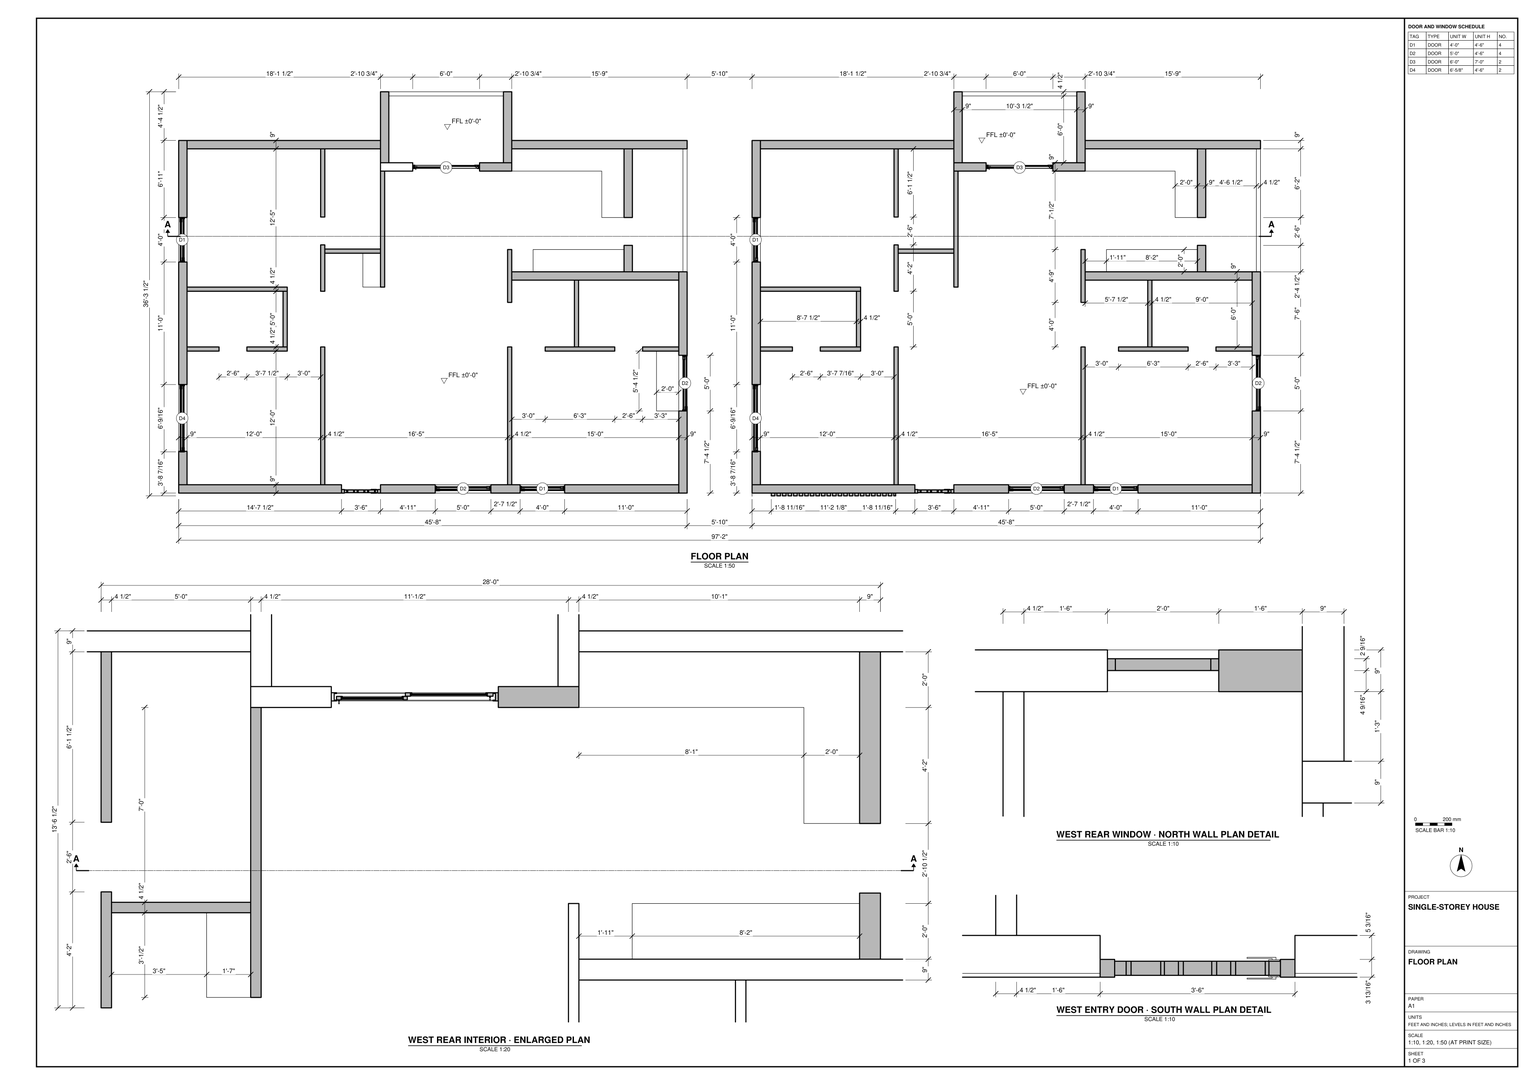
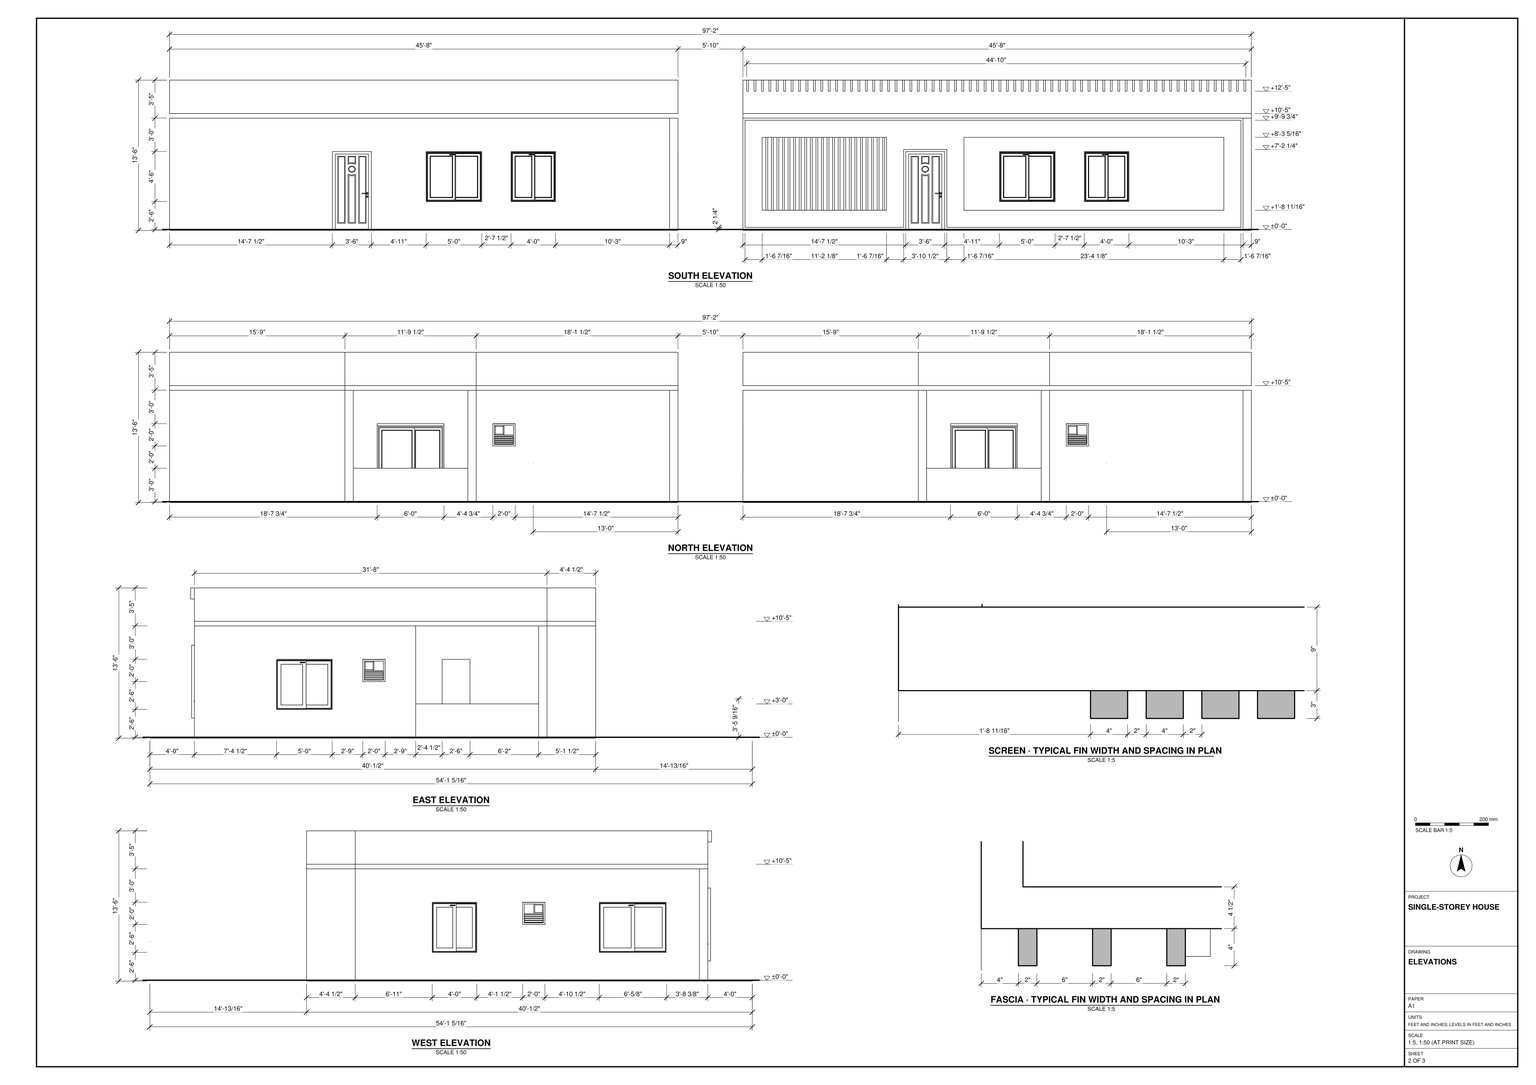
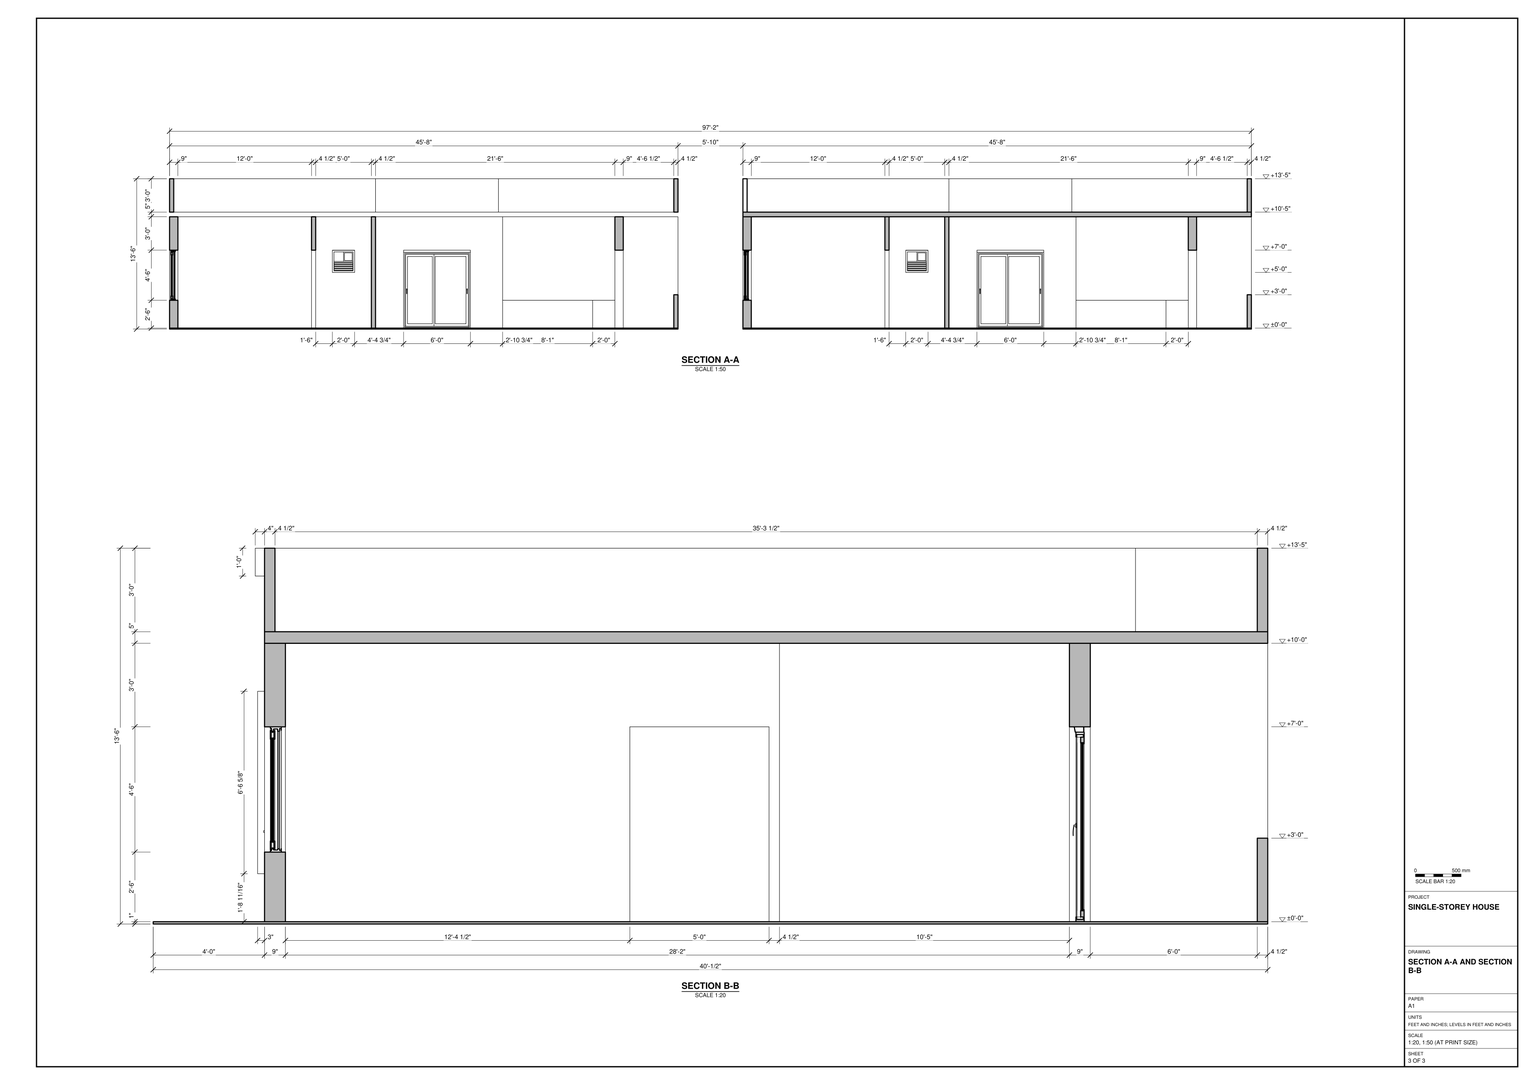
Build a SketchUp model from task_files/diagram_01.pdf. Work in feet and inches. Set the finished floor of both blocks at ±0'-0". The overall model extents are 97'-2" east to west, 54'-1 5/16" north to south and 13'-6" vertically.

Lay out the blocks side by side with their entrances facing south. Each block is 45'-8" wide, with a 5'-10" clear gap between them. Follow the floor plan for the exterior walls, thinner interior partitions, passages and projecting rear bays. Use the enlarged rear plan to place the built-in work surfaces and their returns. Model the floor slabs, flat roof and parapets as shown in section.

Fit the entry doors, framed windows, rear sliding doors and small ventilators at the positions and heights shown. Keep the western block's south elevation plain. On the eastern block, model the screen to the left of the entrance, the surround at the pair of windows and the fins along the fascia. Use the separate plan details for the screen and fascia rather than giving both the same spacing.

Keep shell elements such as walls, slabs and roof, and each furniture or joinery piece, in separate groups or components. Use components for repeated parts. Decor and loose items may be any suitable library components. Save one SketchUp model as output_files/two_single_storey_house_blocks_with_distinct_facades.skp.

# SketchUp Ruby script. Lengths in inches.
U = 1.inch
M = Sketchup.active_model
def pt(a) = Geom::Point3d.new(a.map { |v| v * U })
def face(e, loops, mat)
  f = e.add_face(loops[0].map { |a| pt(a) })
  loops[1..].each { |l| e.add_face(l.map { |a| pt(a) }).erase! }
  f.material = f.back_material = mat if mat
  f
end
# faces: each face lists its corners as indices into pts; further lists are holes
def faces(e, pts, list, mat = nil) = list.each { |f| face(e, (f[0].is_a?(Array) ? f : [f]).map { |l| l.map { |i| pts[i] } }, mat) }
# xy, xz, yz: faces in a plane at the given z, y or x. An outline is a flat list of corners, or four numbers for a rectangle; further outlines are holes
def ring(l) = l.size == 4 ? [[l[0], l[1]], [l[2], l[1]], [l[2], l[3]], [l[0], l[3]]] : l.each_slice(2).to_a
def flat(e, list, mat, &to3) = list.each { |f| face(e, (f[0].is_a?(Array) ? f : [f]).map { |l| ring(l).map { |u, v| to3.(u, v) } }, mat) }
def xy(e, z, list, mat = nil) = flat(e, list, mat) { |x, y| [x, y, z] }
def xz(e, y, list, mat = nil) = flat(e, list, mat) { |x, z| [x, y, z] }
def yz(e, x, list, mat = nil) = flat(e, list, mat) { |y, z| [x, y, z] }
def lines(e, pts, list) = list.each { |a, b| e.add_line(pt(pts[a]), pt(pts[b])) }
# prism: a flat outline (further loops are holes) pulled along v
def prism(e, loops, v, mat = nil)
  f = face(e, loops, mat); d = Geom::Vector3d.new(v.map { |x| x * U })
  f.pushpull(f.normal.samedirection?(d) ? d.length : -d.length)
end
def box(e, o, s, mat = nil) = prism(e, [[o, [o[0] + s[0], o[1], o[2]], [o[0] + s[0], o[1] + s[1], o[2]], [o[0], o[1] + s[1], o[2]]]], [0, 0, s[2]], mat)
def at(x, y, z, deg = 0) = Geom::Transformation.translation(pt([x, y, z])) * Geom::Transformation.rotation(ORIGIN, Z_AXIS, deg.degrees)
def axes(o, x, y, z) = Geom::Transformation.new([*x, 0, *y, 0, *z, 0, *pt(o).to_a, 1])
def part(name) = M.definitions.add(name)
# library, detail: a bought-in or finely detailed component or shape, given as its bounding box
def library(name, o, s) = part(name).tap { |d| box(d.entities, o, s) }
def detail(e, o, s) = box(e.add_group.entities, o, s)
def put(e, d, t, mat = nil) = e.add_instance(d, t).tap { |i| i.material = mat if mat }
def group(e, t, mat = nil) = e.add_group.tap { |g| g.transformation = t; g.material = mat if mat }.entities
root = M.entities
M.materials.add("H01_Misty_Ice").color = [204, 255, 255]
M.materials.add("M04_Stone_Frost").color = [142, 142, 142]
M.materials.add("M06_Steel_Smoke").color = [86, 86, 86]
M.materials.add("Plywood_01_1K").color = [125, 96, 64]
M.materials.add("[Carpet_Plush_Charcoal]").color = [87, 87, 87]
c1 = library("FLOOR PLAN.dwg",[0,0,0],[575,432.5,0.01])
c2 = library("AS-120-mm",[0,0,0],[48,4.72,54])
c3 = library("AS-120-mm\#1",[0,0,0],[60,4.72,54])
c4 = library("door58",[0,0,0],[34.0625,4.69,78.29])
c5 = library("AS-120-mm\#2",[0,0,0],[72.6,4.72,54])
c6 = library("AS-120-mm\#3",[0,0,0],[48,4.72,54])
c7 = library("UPVC DOOR",[0,0,0],[70.79,4.86,80.97])
c8 = library("A.RAJAGANESH",[-0.0625,0,0],[88.9,9.87,1])
c9 = part("Group\#2")
prism(c9.entities,[[[0,371,0],[0,0,0],[0,0,120],[0,371,120]],[[0,36,84],[0,36,30],[0,108,30],[0,108,84]],[[0,240,30],[0,288,30],[0,288,84],[0,240,84]],[[0,166.5,60],[0,190.5,60],[0,190.5,84],[0,166.5,84]]],[9,0,0])
c10 = part("Group\#3")
prism(c10.entities,[[[208.5,9,0],[0,9,0],[0,9,120],[208.5,9,120]],[[190.5,9,84],[166.5,9,84],[166.5,9,60],[190.5,9,60]]],[0,-9,0])
c11 = part("Group\#4")
box(c11.entities,[0,0,0],[9,76.5,120])
c12 = part("Group\#5")
prism(c12.entities,[[[0,0,0],[34.75,0,0],[34.75,0,84],[106.75,0,84],[106.75,0,0],[141.5,0,0],[141.5,0,120],[0,0,120]]],[0,9,0])
c13 = part("Group\#6")
box(c13.entities,[0,0,0],[9,76.5,120])
c14 = part("Group\#7")
box(c14.entities,[0,0,0],[189,9,120])
c15 = part("Group\#8")
prism(c15.entities,[[[0,132.52,0],[0,58.5,0],[0,58.5,84],[0,28.5,84],[0,28.5,0],[0,0,0],[0,0,120],[0,132.52,120]]],[9,0,0])
c16 = part("Group\#9")
box(c16.entities,[0,0,0],[180,8.98,120.04])
c17 = part("Group\#11")
box(c17.entities,[0,0,0],[4.5,132.52,36])
c18 = library("Group\#275",[0,0,0],[28,3,28])
c19 = part("Group\#17")
prism(c19.entities,[[[108,4.5,0],[0,4.5,0],[0,4.5,120],[144,4.5,120],[144,4.5,84],[108,4.5,84]]],[0,-4.5,0])
c20 = part("Group\#18")
prism(c20.entities,[[[0,0,0],[34.5,0,0],[34.5,0,84],[64.5,0,84],[64.5,0,0],[108,0,0],[108,0,84],[144,0,84],[144,0,120],[0,0,120]]],[0,4.5,0])
c21 = part("Group\#20")
box(c21.entities,[0,0,0],[4.5,60,120])
c22 = part("Group\#21")
prism(c22.entities,[[[0,148.5,0],[0,0,0],[0,0,120],[0,362,120],[0,362,0],[0,288.5,0],[0,288.5,84],[0,258.5,84],[0,258.5,0],[0,208.5,0],[0,208.5,84],[0,148.5,84]]],[4.5,0,0])
c23 = part("Group\#22")
box(c23.entities,[0,0,0],[4.5,125,120])
c24 = part("Group\#23")
box(c24.entities,[0,0,0],[60,4.5,120])
c25 = part("Group\#24")
box(c25.entities,[0,0,0],[4.5,72,120])
c26 = part("Group\#25")
box(c26.entities,[0,0,0],[4.5,148.5,120])
c27 = part("Group\#26")
prism(c27.entities,[[[141,0,0],[180,0,0],[180,0,120],[0,0,120],[0,0,84],[36,0,84],[36,0,0],[111,0,0],[111,0,84],[141,0,84]]],[0,4.5,0])
c28 = part("Group\#28")
box(c28.entities,[0,0,0],[4.5,56.98,120])
c29 = part("Group\#30")
prism(c29.entities,[[[97,50.02,0],[0,50.02,0],[0,74.02,0],[121,74.02,0],[121,0,0],[97,0,0]]],[0,0,30])
c30 = part("Component\#1")
box(c30.entities,[0,-4,0],[2,4,12])
c31 = part("Group125\#1")
box(c31.entities,[-67.06,-39.31,0],[4,78.62,3])
c32 = part("Group126\#1")
box(c32.entities,[-61.06,-39.31,0],[4,78.62,3])
c33 = part("Group127\#1")
box(c33.entities,[-55.06,-39.31,0],[4,78.62,3])
c34 = part("Group128\#1")
box(c34.entities,[-49.06,-39.31,0],[4,78.62,3])
c35 = part("Group129\#1")
box(c35.entities,[-43.06,-39.31,0],[4,78.62,3])
c36 = part("Group130\#1")
box(c36.entities,[-37.06,-39.31,0],[4,78.62,3])
c37 = part("Group131\#1")
box(c37.entities,[-31.06,-39.31,0],[4,78.62,3])
c38 = part("Group132\#1")
box(c38.entities,[-25.06,-39.31,0],[4,78.62,3])
c39 = part("Group133\#1")
box(c39.entities,[-19.06,-39.31,0],[4,78.62,3])
c40 = part("Group134\#1")
box(c40.entities,[-13.06,-39.31,0],[4,78.62,3])
c41 = part("Group135\#1")
box(c41.entities,[-7.06,-39.31,0],[4,78.62,3])
c42 = part("Group136\#1")
box(c42.entities,[-1.06,-39.31,0],[4,78.62,3])
c43 = part("Group137\#1")
box(c43.entities,[4.94,-39.31,0],[4,78.62,3])
c44 = part("Group138\#1")
box(c44.entities,[10.94,-39.31,0],[4,78.62,3])
c45 = part("Group139\#1")
box(c45.entities,[16.94,-39.31,0],[4,78.62,3])
c46 = part("Group140\#1")
box(c46.entities,[22.94,-39.31,0],[4,78.62,3])
c47 = part("Group141\#1")
box(c47.entities,[28.94,-39.31,0],[4,78.62,3])
c48 = part("Group142\#1")
box(c48.entities,[34.94,-39.31,0],[4,78.62,3])
c49 = part("Group143\#1")
box(c49.entities,[40.94,-39.31,0],[4,78.62,3])
c50 = part("Group144\#1")
box(c50.entities,[46.94,-39.31,0],[4,78.62,3])
c51 = part("Group145\#1")
box(c51.entities,[52.94,-39.31,0],[4,78.62,3])
c52 = part("Group146\#1")
box(c52.entities,[58.94,-39.31,0],[4,78.62,3])
c53 = part("Group147\#1")
box(c53.entities,[64.94,-39.31,0],[2.12,78.62,3])
c54 = part("Group123\#1")
put(c54.entities,c31,at(0,0,0))
put(c54.entities,c32,at(0,0,0))
put(c54.entities,c33,at(0,0,0))
put(c54.entities,c34,at(0,0,0))
put(c54.entities,c35,at(0,0,0))
put(c54.entities,c36,at(0,0,0))
put(c54.entities,c37,at(0,0,0))
put(c54.entities,c38,at(0,0,0))
put(c54.entities,c39,at(0,0,0))
put(c54.entities,c40,at(0,0,0))
put(c54.entities,c41,at(0,0,0))
put(c54.entities,c42,at(0,0,0))
put(c54.entities,c43,at(0,0,0))
put(c54.entities,c44,at(0,0,0))
put(c54.entities,c45,at(0,0,0))
put(c54.entities,c46,at(0,0,0))
put(c54.entities,c47,at(0,0,0))
put(c54.entities,c48,at(0,0,0))
put(c54.entities,c49,at(0,0,0))
put(c54.entities,c50,at(0,0,0))
put(c54.entities,c51,at(0,0,0))
put(c54.entities,c52,at(0,0,0))
put(c54.entities,c53,at(0,0,0))
xy(root,0,[[199.5,270,199.5,287.54,200.5,287.54,200.5,288.25,199.5,288.25,199.5,306.5,217.5,306.5,217.5,270]])
xy(root,28,[[198.5,270,199.5,287.54],[198.5,287.54,200.5,288.25],[198.5,288.25,199.5,306.5]])
xy(root,30,[[198.5,270,217.5,306.5]])
xz(root,270,[[199.5,0,217.5,28],[198.5,28,217.5,30]])
xz(root,287.54,[[199.5,0,200.5,28]])
xz(root,288.25,[[199.5,0,200.5,28]])
xz(root,306.5,[[199.5,0,199.5,28,198.5,28,198.5,30,217.5,30,217.5,0]])
yz(root,198.5,[[270,28,306.5,30]])
yz(root,199.5,[[270,0,287.54,28],[288.25,0,306.5,28]])
yz(root,200.5,[[287.54,0,288.25,28]])
yz(root,217.5,[[270,0,306.5,30]])
put(root,c1,at(-27,48,0))
put(root,c2,at(368,50.5,30))
put(root,c3,at(276.5,50.5,30))
put(root,c4,axes([217.5,47.59,0],[-1.233,0,0],[0,1,0],[0,0,1.07289]))
put(root,c5,at(1.4,165,30,-90))
put(root,c6,at(1.4,345,30,-90))
put(root,c3,at(548,136.5,30,90))
put(root,c7,axes([252.25,396.49,0],[1.01713,0,0],[0,1,0],[0,0,1.03744]))
put(root,c8,axes([155.97,649.32,41.52],[0,-0.00219,0],[0,0,0.00219],[-0.00219,0,0]),"[Carpet_Plush_Charcoal]")
put(root,c1,at(590.98,48,0))
put(root,c2,at(985.98,50.5,30))
put(root,c3,at(894.48,50.5,30))
put(root,c6,at(619.38,345,30,-90))
put(root,c7,axes([870.23,396.49,0],[1.01713,0,0],[0,1,0],[0,0,1.03744]))
put(root,c8,axes([773.96,649.32,41.52],[0,-0.00219,0],[0,0,0.00219],[-0.00219,0,0]),"[Carpet_Plush_Charcoal]")
put(root,c5,at(619.38,165,30,-90))
put(root,c4,axes([835.48,47.59,0],[-1.233,0,0],[0,1,0],[0,0,1.07289]))
put(root,c3,at(1165.98,136.5,30,90))
g1 = group(root,at(0,48,0))
prism(g1,[[[539,9,0],[217.5,9,0],[217.5,9,84],[175.5,9,84],[175.5,9,0],[0,9,0],[0,9,120],[539,9,120]],[[336.5,9,30],[336.5,9,84],[276.5,9,84],[276.5,9,30]],[[368,9,30],[416,9,30],[416,9,84],[368,9,84]]],[0,-9,0])
put(root,c9,at(0,57,0))
put(root,c10,at(9,419,0))
put(root,c11,at(217.5,404,0))
put(root,c12,at(217.5,395,0))
put(root,c13,at(350,404,0))
put(root,c14,at(359,419,0))
put(root,c15,at(480,286.48,0))
put(root,c16,at(359,277.5,-0.04))
g2 = group(root,at(539,48,0))
prism(g2,[[[0,238.48,0],[0,0,0],[0,0,120],[0,238.48,120]],[[0,148.5,30],[0,148.5,84],[0,88.5,84],[0,88.5,30]],[[0,205.5,84],[0,181.5,84],[0,181.5,60],[0,205.5,60]]],[9,0,0])
put(root,c17,at(543.5,286.48,0))
g3 = group(root,at(0,48,-1))
xy(g3,0,[[0,0.82,0,380,217.5,380,217.5,432.5,359,432.5,359,380,548,380,548,0.82]])
xy(g3,1,[[0,0.82,548,0.82,548,380,359,380,359,432.5,350,432.5,350,428,226.5,428,226.5,432.5,217.5,432.5,217.5,380,0,380],[226.5,428,350,432.5]])
xy(g3,37,[[226.5,428,350,432.5]])
xz(g3,0.82,[[0,0,548,1]])
xz(g3,380,[[0,0,217.5,1],[359,0,548,1]])
xz(g3,428,[[226.5,1,350,37]])
xz(g3,432.5,[[217.5,0,226.5,1],[226.5,0,350,1],[350,0,359,1],[226.5,1,350,37]])
yz(g3,0,[[0.82,0,380,1]])
yz(g3,217.5,[[380,0,432.5,1]])
yz(g3,226.5,[[428,1,432.5,37]])
yz(g3,350,[[428,1,432.5,37]])
yz(g3,359,[[380,0,432.5,1]])
yz(g3,548,[[0.82,0,380,1]])
put(root,c18,axes([175.5,423.55,60],[0.85714,0,0],[0,0.85,0],[0,0,0.85]))
put(root,c18,axes([543.73,253.5,60],[0,-0.85714,0],[0.85,0,0],[0,0,0.85]))
put(root,c18,axes([1.48,247.5,60],[0,-0.85714,0],[0.85,0,0],[0,0,0.85]))
put(root,c19,at(9,265.5,0))
put(root,c20,at(9,201,0))
put(root,c21,at(112.5,205.5,0))
put(root,c22,at(153,57,0))
put(root,c23,at(217.5,270,0))
put(root,c24,at(157.5,306.5,0))
put(root,c25,at(426.5,205.5,0))
put(root,c26,at(354.5,57,0))
put(root,c27,at(359,201,0))
put(root,c28,at(354.5,253.5,0))
put(root,c29,at(359,344.98,0))
g4 = group(root,at(381.98,286.48,0))
box(g4,[0,0,0],[98.02,24,30])
g5 = group(root,at(0,48,125))
prism(g5,[[[359,432.5,0],[359,380,0],[548,380,0],[548,0,0],[0,0,0],[0,380,0],[217.5,380,0],[217.5,432.5,0]],[[354.5,428,0],[222,428,0],[222,375.5,0],[4.5,375.5,0],[4.5,4.5,0],[543.5,4.5,0],[543.5,375.5,0],[354.5,375.5,0]]],[0,0,36])
put(root,c13,at(967.98,404,0))
put(root,c28,at(972.48,253.5,0))
put(root,c9,at(617.98,57,0))
put(root,c27,at(976.98,201,0))
g6 = group(root,at(617.98,48,-1))
xy(g6,0,[[0,-48,0,380,217.5,380,217.5,432.5,359,432.5,359,380,548,380,548,-48]])
xy(g6,1,[[0,-48,548,-48,548,380,359,380,359,432.5,350,432.5,350,428,226.5,428,226.5,432.5,217.5,432.5,217.5,380,0,380],[226.5,428,350,432.5]])
xy(g6,37,[[226.5,428,350,432.5]])
xz(g6,-48,[[0,0,548,1]])
xz(g6,380,[[0,0,217.5,1],[359,0,548,1]])
xz(g6,428,[[226.5,1,350,37]])
xz(g6,432.5,[[217.5,0,226.5,1],[226.5,0,350,1],[350,0,359,1],[226.5,1,350,37]])
yz(g6,0,[[-48,0,380,1]])
yz(g6,217.5,[[380,0,432.5,1]])
yz(g6,226.5,[[428,1,432.5,37]])
yz(g6,350,[[428,1,432.5,37]])
yz(g6,359,[[380,0,432.5,1]])
yz(g6,548,[[-48,0,380,1]])
put(root,c23,at(835.48,270,0))
g7 = group(root,at(617.98,48,120),"M06_Steel_Smoke")
xy(g7,0,[[0,0,0,380,217.5,380,217.5,432.5,359,432.5,359,380,548,380,548,0]])
xy(g7,5,[[[0,0,548,0,548,380,359,380,359,432.5,217.5,432.5,217.5,380,0,380],[4.5,4.5,4.5,375.5,222,375.5,222,428,354.5,428,354.5,375.5,543.5,375.5,543.5,4.5]],[4.5,4.5,543.5,4.5,543.5,375.5,354.5,375.5,354.5,428,222,428,222,375.5,4.5,375.5]])
xz(g7,0,[[0,0,548,5]])
xz(g7,380,[[0,0,217.5,5],[359,0,548,5]])
xz(g7,432.5,[[217.5,0,359,5]])
yz(g7,0,[[0,0,380,5]])
yz(g7,217.5,[[380,0,432.5,5]])
yz(g7,359,[[380,0,432.5,5]])
yz(g7,548,[[0,0,380,5]])
put(root,c12,at(835.48,395,0))
g8 = group(root,at(617.98,48,125))
xy(g8,0,[[[0,0,0,380,217.5,380,217.5,432.5,359,432.5,359,380,548,380,548,0],[4.5,4.5,543.5,4.5,543.5,375.5,354.5,375.5,354.5,428,222,428,222,375.5,4.5,375.5]]])
xy(g8,36,[[[0,0,548,0,548,380,359,380,359,432.5,217.5,432.5,217.5,380,0,380],[4.5,4.5,4.5,375.5,222,375.5,222,428,354.5,428,354.5,375.5,543.5,375.5,543.5,4.5]]])
xz(g8,0,[[0,0,548,36]],"M06_Steel_Smoke")
xz(g8,4.5,[[4.5,0,543.5,36]])
xz(g8,375.5,[[4.5,0,222,36],[354.5,0,543.5,36]])
xz(g8,380,[[0,0,217.5,36],[359,0,548,36]])
xz(g8,428,[[222,0,354.5,36]])
xz(g8,432.5,[[217.5,0,359,36]])
yz(g8,0,[[0,0,380,36]])
yz(g8,4.5,[[4.5,0,375.5,36]])
yz(g8,217.5,[[380,0,432.5,36]])
yz(g8,222,[[375.5,0,428,36]])
yz(g8,354.5,[[375.5,0,428,36]])
yz(g8,359,[[380,0,432.5,36]])
yz(g8,543.5,[[4.5,0,375.5,36]])
yz(g8,548,[[0,0,380,36]])
put(root,c29,at(976.98,344.98,0))
put(root,c11,at(835.48,404,0))
put(root,c10,at(626.98,419,0))
g9 = group(root,at(617.98,48,0),"M06_Steel_Smoke")
xy(g9,0,[[0,0,175.5,9],[217.5,0,539,9]])
xy(g9,30,[[276.5,0,336.5,9],[368,0,416,9]])
xy(g9,84,[[175.5,0,217.5,9],[276.5,0,336.5,9],[368,0,416,9]])
xy(g9,120,[[0,0,539,9]])
xz(g9,0,[[[0,0,175.5,0,175.5,84,217.5,84,217.5,0,539,0,539,120,0,120],[2.26,2.26,2.26,117.74,536.74,117.74,536.74,2.26,219.76,2.26,219.76,86.26,173.24,86.26,173.24,2.26]]])
xz(g9,0,[[[238.19,20.69,518.31,99.31],[276.5,30,336.5,84],[368,30,416,84]]],"H01_Misty_Ice")
xz(g9,0,[[[2.26,2.26,173.24,2.26,173.24,86.26,219.76,86.26,219.76,2.26,536.74,2.26,536.74,117.74,2.26,117.74],[238.19,20.69,518.31,99.31],[20.69,20.69,154.81,99.31]],[20.69,20.69,154.81,99.31]],"M04_Stone_Frost")
xz(g9,9,[[[0,0,0,120,539,120,539,0,217.5,0,217.5,84,175.5,84,175.5,0],[276.5,30,336.5,84],[368,30,416,84]]])
yz(g9,0,[[0,0,9,120]])
yz(g9,175.5,[[0,0,9,84]])
yz(g9,217.5,[[0,0,9,84]])
yz(g9,276.5,[[0,30,9,84]])
yz(g9,336.5,[[0,30,9,84]])
yz(g9,368,[[0,30,9,84]])
yz(g9,416,[[0,30,9,84]])
yz(g9,539,[[0,0,9,120]])
put(root,c18,axes([1161.72,253.5,60],[0,-0.85714,0],[0.85,0,0],[0,0,0.85]))
put(root,c22,at(770.98,57,0))
g10 = group(root,at(999.96,286.48,0))
box(g10,[0,0,0],[98.02,24,24])
put(root,c18,axes([793.48,423.55,60],[0.85714,0,0],[0,0.85,0],[0,0,0.85]))
put(root,c21,at(730.48,205.5,0))
put(root,c26,at(972.48,57,0))
put(root,c25,at(1044.48,205.5,0))
put(root,c20,at(626.98,201,0))
put(root,c24,at(775.48,306.5,0))
put(root,c14,at(976.98,419,0))
g11 = group(root,at(1149.98,48,149))
put(g11,c30,at(8,0,0))
put(g11,c30,at(0,0,0))
put(g11,c30,at(-8,0,0))
put(g11,c30,at(-16,0,0))
put(g11,c30,at(-24,0,0))
put(g11,c30,at(-32,0,0))
put(g11,c30,at(-40,0,0))
put(g11,c30,at(-48,0,0))
put(g11,c30,at(-56,0,0))
put(g11,c30,at(-64,0,0))
put(g11,c30,at(-72,0,0))
put(g11,c30,at(-80,0,0))
put(g11,c30,at(-88,0,0))
put(g11,c30,at(-96,0,0))
put(g11,c30,at(-104,0,0))
put(g11,c30,at(-112,0,0))
put(g11,c30,at(-120,0,0))
put(g11,c30,at(-128,0,0))
put(g11,c30,at(-136,0,0))
put(g11,c30,at(-144,0,0))
put(g11,c30,at(-152,0,0))
put(g11,c30,at(-160,0,0))
put(g11,c30,at(-168,0,0))
put(g11,c30,at(-176,0,0))
put(g11,c30,at(-184,0,0))
put(g11,c30,at(-192,0,0))
put(g11,c30,at(-200,0,0))
put(g11,c30,at(-208,0,0))
put(g11,c30,at(-216,0,0))
put(g11,c30,at(-224,0,0))
put(g11,c30,at(-232,0,0))
put(g11,c30,at(-240,0,0))
put(g11,c30,at(-248,0,0))
put(g11,c30,at(-256,0,0))
put(g11,c30,at(-264,0,0))
put(g11,c30,at(-272,0,0))
put(g11,c30,at(-280,0,0))
put(g11,c30,at(-288,0,0))
put(g11,c30,at(-296,0,0))
put(g11,c30,at(-304,0,0))
put(g11,c30,at(-312,0,0))
put(g11,c30,at(-320,0,0))
put(g11,c30,at(-328,0,0))
put(g11,c30,at(-336,0,0))
put(g11,c30,at(-344,0,0))
put(g11,c30,at(-352,0,0))
put(g11,c30,at(-360,0,0))
put(g11,c30,at(-368,0,0))
put(g11,c30,at(-376,0,0))
put(g11,c30,at(-384,0,0))
put(g11,c30,at(-392,0,0))
put(g11,c30,at(-400,0,0))
put(g11,c30,at(-408,0,0))
put(g11,c30,at(-416,0,0))
put(g11,c30,at(-424,0,0))
put(g11,c30,at(-432,0,0))
put(g11,c30,at(-440,0,0))
put(g11,c30,at(-448,0,0))
put(g11,c30,at(-456,0,0))
put(g11,c30,at(-464,0,0))
put(g11,c30,at(-472,0,0))
put(g11,c30,at(-480,0,0))
put(g11,c30,at(-488,0,0))
put(g11,c30,at(-496,0,0))
put(g11,c30,at(-504,0,0))
put(g11,c30,at(-512,0,0))
put(g11,c30,at(-520,0,0))
put(g11,c30,at(-528,0,0))
put(root,c15,at(1097.98,286.48,0))
put(root,c19,at(626.98,265.5,0))
put(root,c18,axes([619.46,247.5,60],[0,-0.85714,0],[0.85,0,0],[0,0,0.85]))
put(root,c16,at(976.98,277.5,-0.04))
put(root,c54,axes([705.73,48,60],[1,0,0],[0,0,1],[0,-1,0]),"Plywood_01_1K")
g12 = group(root,at(1156.98,48,0))
xy(g12,0,[[0,0,9,238.48]])
xy(g12,30,[[0,88.5,9,148.5]])
xy(g12,60,[[0,181.5,9,205.5]])
xy(g12,84,[[0,88.5,9,148.5],[0,181.5,9,205.5]])
xy(g12,120,[[0,0,9,238.48]])
xz(g12,0,[[0,0,9,120]],"M06_Steel_Smoke")
xz(g12,88.5,[[0,30,9,84]])
xz(g12,148.5,[[0,30,9,84]])
xz(g12,181.5,[[0,60,9,84]])
xz(g12,205.5,[[0,60,9,84]])
xz(g12,238.48,[[0,0,9,120]])
yz(g12,0,[[[0,0,238.48,120],[88.5,30,148.5,84],[181.5,60,205.5,84]]])
yz(g12,9,[[[0,0,238.48,120],[88.5,30,148.5,84],[181.5,60,205.5,84]]])
put(root,c17,at(1161.48,286.48,0))
g13 = group(root,at(515,136.5,0))
box(g13,[0,0,0],[24,64.5,24])
